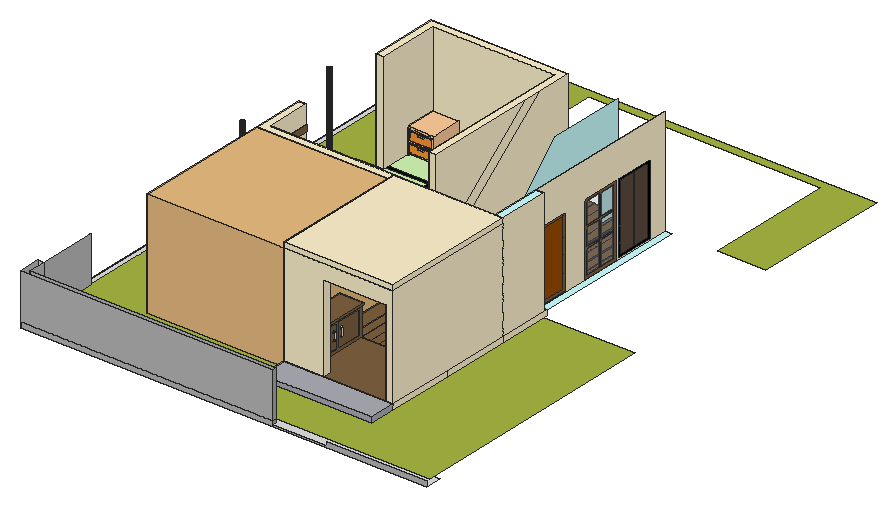
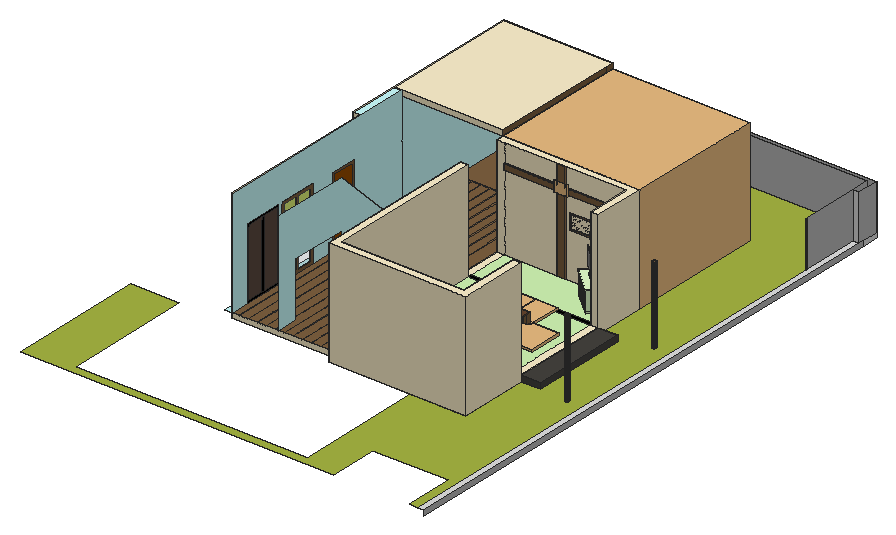
# SketchUp Ruby script. Lengths in inches.
U = 1.inch
M = Sketchup.active_model
def pt(a) = Geom::Point3d.new(a.map { |v| v * U })
def face(e, loops, mat)
  f = e.add_face(loops[0].map { |a| pt(a) })
  loops[1..].each { |l| e.add_face(l.map { |a| pt(a) }).erase! }
  f.material = f.back_material = mat if mat
  f
end
# faces: each face lists its corners as indices into pts; further lists are holes
def faces(e, pts, list, mat = nil) = list.each { |f| face(e, (f[0].is_a?(Array) ? f : [f]).map { |l| l.map { |i| pts[i] } }, mat) }
# xy, xz, yz: faces in a plane at the given z, y or x. An outline is a flat list of corners, or four numbers for a rectangle; further outlines are holes
def ring(l) = l.size == 4 ? [[l[0], l[1]], [l[2], l[1]], [l[2], l[3]], [l[0], l[3]]] : l.each_slice(2).to_a
def flat(e, list, mat, &to3) = list.each { |f| face(e, (f[0].is_a?(Array) ? f : [f]).map { |l| ring(l).map { |u, v| to3.(u, v) } }, mat) }
def xy(e, z, list, mat = nil) = flat(e, list, mat) { |x, y| [x, y, z] }
def xz(e, y, list, mat = nil) = flat(e, list, mat) { |x, z| [x, y, z] }
def yz(e, x, list, mat = nil) = flat(e, list, mat) { |y, z| [x, y, z] }
def lines(e, pts, list) = list.each { |a, b| e.add_line(pt(pts[a]), pt(pts[b])) }
# prism: a flat outline (further loops are holes) pulled along v
def prism(e, loops, v, mat = nil)
  f = face(e, loops, mat); d = Geom::Vector3d.new(v.map { |x| x * U })
  f.pushpull(f.normal.samedirection?(d) ? d.length : -d.length)
end
def box(e, o, s, mat = nil) = prism(e, [[o, [o[0] + s[0], o[1], o[2]], [o[0] + s[0], o[1] + s[1], o[2]], [o[0], o[1] + s[1], o[2]]]], [0, 0, s[2]], mat)
def at(x, y, z, deg = 0) = Geom::Transformation.translation(pt([x, y, z])) * Geom::Transformation.rotation(ORIGIN, Z_AXIS, deg.degrees)
def axes(o, x, y, z) = Geom::Transformation.new([*x, 0, *y, 0, *z, 0, *pt(o).to_a, 1])
def part(name) = M.definitions.add(name)
# library, detail: a bought-in or finely detailed component or shape, given as its bounding box
def library(name, o, s) = part(name).tap { |d| box(d.entities, o, s) }
def detail(e, o, s) = box(e.add_group.entities, o, s)
def put(e, d, t, mat = nil) = e.add_instance(d, t).tap { |i| i.material = mat if mat }
def group(e, t, mat = nil) = e.add_group.tap { |g| g.transformation = t; g.material = mat if mat }.entities
root = M.entities
M.materials.add("A02_Rose_Quartz").color = [255, 153, 153]
M.materials.add("A04_Scarlet_Glow").color = [255, 49, 49]
M.materials.add("Black_Lines_1_1K").color = [210, 247, 181]
M.materials.add("Brick_Stack_Bond_2K2").color = [186, 186, 186]
M.materials.add("C02_Golden_Beige").color = [255, 205, 155]
M.materials.add("C04_Amber_Sunshine").color = [255, 152, 49]
M.materials.add("C07_Caramel_Shine").color = [153, 76, 0]
M.materials.add("D01_Frost_White").color = [255, 242, 206]
M.materials.add("F01_Seafoam_Drift").color = [229, 255, 204]
M.materials.add("Fabric_13_1K").color = [243, 117, 128]
M.materials["Fabric_13_1K"].alpha = 0.97
M.materials.add("Glass_Basic_1").color = [161, 173, 186]
M.materials["Glass_Basic_1"].alpha = 0.25
M.materials.add("Glass_Mirror_01").color = [185, 185, 185]
M.materials["Glass_Mirror_01"].alpha = 0.58
M.materials.add("H01_Misty_Ice1").color = [204, 255, 255]
M.materials.add("M00_Soft_Cloud").color = [255, 255, 255]
M.materials.add("M01_Silver_Fog").color = [224, 224, 224]
M.materials.add("M03_Pewter_Shine").color = [168, 168, 168]
M.materials.add("M04_Stone_Frost").color = [142, 142, 142]
M.materials.add("M07_Charcoal_Gleam").color = [58, 58, 58]
M.materials.add("M09_Shadow_Night").color = [0, 0, 0]
M.materials.add("Marble_20_1K").color = [172, 173, 182]
M.materials.add("Metal_06_1K").color = [238, 236, 231]
M.materials.add("Metal_10_1K").color = [196, 175, 123]
M.materials.add("Plywood_01_1K").color = [125, 96, 64]
M.materials.add("Soil_04_1K").color = [167, 182, 67]
M.materials.add("Wood_Floor_01_1K1").color = [146, 111, 76]
M.materials.add("Wood_Floor_12_1K").color = [92, 75, 65]
M.materials.add("Wood_Planks_01_1K1").color = [69, 67, 63]
M.materials.add("Wood_Veneer_15_1K").color = [103, 69, 45]
c1 = part("Group\#52")
box(c1.entities,[0,0,0],[1.5,12,12.52])
c2 = library("Group\#7",[0,0,0],[162,162,126])
c3 = library("Group\#106",[0,0,0],[9.9375,0.625,10.1875])
c4 = part("Group\#101")
box(c4.entities,[0,0,0],[6,6,17.625],"Plywood_01_1K")
c5 = library("Group\#105",[0,0,-6.9375],[37.03,37.03,8.9375])
c6 = part("Group\#134")
box(c6.entities,[0,0,0],[10.25,2.1875,0.25],"Metal_10_1K")
c7 = library("Group\#86",[-0.0625,-4,0],[20.0625,57.25,28.48])
c8 = part("Group\#46")
detail(c8.entities,[0,0,0],[3.47,3.07,3.07])
c9 = part("Group\#153")
xy(c9.entities,0,[[0,-9.8125,1.5625,-7.9375],[0,-0.1875,1.5625,0],[0,0,1.5625,1.5625]],"Metal_06_1K")
xy(c9.entities,0.29,[[0,-9.8125,1.5625,-8.1875]],"Metal_06_1K")
xy(c9.entities,0.3125,[[0,0,1.5625,1.5625]],"Metal_06_1K")
xy(c9.entities,2.125,[[0,-7.9375,1.5625,-0.1875],[0,-0.1875,1.5625,0]],"Metal_06_1K")
xy(c9.entities,2.375,[[0,-8.1875,1.5625,-7.9375],[0,-7.9375,1.5625,0]],"Metal_06_1K")
xz(c9.entities,-9.8125,[[0,0,1.5625,0.29]],"Metal_06_1K")
xz(c9.entities,-8.1875,[[0,0.29,1.5625,2.375]],"Metal_06_1K")
xz(c9.entities,-7.9375,[[0,0,1.5625,2.125],[0,2.125,1.5625,2.375]],"Metal_06_1K")
xz(c9.entities,-0.1875,[[0,0,1.5625,2.125]],"Metal_06_1K")
xz(c9.entities,0,[[0,0,1.5625,0.3125],[0,0.3125,1.5625,2.125],[0,2.125,1.5625,2.375]],"Metal_06_1K")
xz(c9.entities,1.5625,[[0,0,1.5625,0.3125]],"Metal_06_1K")
yz(c9.entities,0,[[-9.8125,0,-9.8125,0.29,-8.1875,0.29,-8.1875,2.375,-7.9375,2.375,-7.9375,0],[-0.1875,0,0,2.125],[0,0,1.5625,0.3125],[-7.9375,2.125,0,2.375]],"Metal_06_1K")
yz(c9.entities,1.5625,[[-9.8125,0,-7.9375,0,-7.9375,2.375,-8.1875,2.375,-8.1875,0.29,-9.8125,0.29],[-0.1875,0,0,2.125],[0,0,1.5625,0.3125],[-7.9375,2.125,0,2.375]],"Metal_06_1K")
xy(root,6,[[1567.75,129.625,2047.75,149.6875]],"M01_Silver_Fog")
xy(root,12,[[1648.75,215.6875,1801.75,215.6875,1801.75,224.6875,1657.75,224.6875,1657.75,368.6875,1648.75,368.6875],[1801.75,215.6875,1810.75,215.6875,1810.75,580.6875,1876.75,580.6875,1876.75,590.6875,1810.75,590.6875,1810.75,635.6875,1657.75,635.6875,1657.75,626.6875,1801.75,626.6875,1801.75,377.6875,1648.75,377.6875,1648.75,368.6875,1801.75,368.6875],[1657.75,224.6875,1801.75,368.6875],[1810.75,224.6875,1930.75,368.6875],[1648.75,377.6875,1657.75,635.6875],
  [1657.75,377.6875,1801.75,626.6875]],"Brick_Stack_Bond_2K2")
xy(root,12,[[1567.75,129.625,1574.75,149.6875],[1574.75,129.625,1865.79,134.375],[1567.75,149.6875,1574.75,155.6875],[1567.75,155.6875,1567.75,798.625,1574.3125,798.625,1574.3125,224.6875,1574.75,224.6875,1574.75,155.6875]],"M01_Silver_Fog")
xy(root,12,[[1574.75,134.375,2047.75,134.375,2047.75,437.6875,1939.75,437.6875,1939.75,215.6875,1648.75,215.6875,1648.75,635.6875,1712.6875,635.6875,1712.6875,788.6875,1986.9375,788.6875,1986.9375,635.6875,2044.5625,635.6875,2044.5625,798.625,1674.5,798.625,1674.5,740.6875,1584.5,740.6875,1584.5,798.625,1574.3125,798.625,1574.3125,224.6875,1574.75,224.6875]],"Soil_04_1K")
xy(root,18,[[1876.75,440.3125,1882.75,533.5]],"Brick_Stack_Bond_2K2")
xy(root,18,[[1876.75,435.3125,1882.75,440.3125]],"Wood_Floor_12_1K")
xz(root,129.625,[[1567.75,6,2047.75,6,2047.75,12,1929.96,12,1929.96,7.5,1865.79,7.5,1865.79,12,1567.75,12],[1567.75,12,1865.79,66]],"Brick_Stack_Bond_2K2")
xz(root,134.375,[[1574.75,12,1865.79,66]],"Brick_Stack_Bond_2K2")
xz(root,155.6875,[[1567.75,12,1574.75,66]],"M01_Silver_Fog")
xz(root,224.6875,[[1574.3125,12,1574.75,66]],"M01_Silver_Fog")
xz(root,435.3125,[[1876.75,18,1882.75,45.8125]],"Wood_Floor_12_1K")
yz(root,1567.75,[[149.6875,6,798.625,12],[129.625,12,155.6875,66]],"Brick_Stack_Bond_2K2")
yz(root,1567.75,[[129.625,6,149.6875,12]],"M01_Silver_Fog")
yz(root,1574.75,[[134.375,12,155.6875,66],[155.6875,12,224.6875,66]],"Brick_Stack_Bond_2K2")
yz(root,1865.79,[[129.625,7.5,134.375,12],[129.625,12,134.375,66]],"M03_Pewter_Shine")
yz(root,1876.75,[[440.3125,18,440.3125,45.8125,533.5,139,626.6875,139,626.6875,18,602.25,18,602.25,82.875,533.5,82.875,533.5,18]],"H01_Misty_Ice1")
yz(root,1876.75,[[435.3125,18,435.3125,45.77,437.79,43.29,440.3125,45.8125,440.3125,18]],"Wood_Floor_12_1K")
g1 = group(root,at(1590.43,424.46,12))
xy(g1,0,[[2.1875,0,1.62,0.07,1.09,0.29,0.64,0.64,0.29,1.09,0.07,1.62,0,2.1875,0.07,2.75,0.29,3.28,0.64,3.73,1.09,4.08,1.62,4.3,2.1875,4.375,2.75,4.3,3.28,4.08,3.73,3.73,4.08,3.28,4.3,2.75,4.375,2.1875,4.3,1.62,4.08,1.09,3.73,0.64,3.28,0.29,2.75,0.07]],"Metal_06_1K")
xy(g1,91.125,[[2.1875,0,2.75,0.07,3.28,0.29,3.73,0.64,4.08,1.09,4.3,1.62,4.375,2.1875,4.3,2.75,4.08,3.28,3.73,3.73,3.28,4.08,2.75,4.3,2.1875,4.375,1.62,4.3,1.09,4.08,0.64,3.73,0.29,3.28,0.07,2.75,0,2.1875,0.07,1.62,0.29,1.09,0.64,0.64,1.09,0.29,1.62,0.07]],"Plywood_01_1K")
p = [[1.62,0.07,0],[2.1875,0,0],[2.1875,0,91.125],[1.62,0.07,91.125],[2.75,0.07,0],[2.75,0.07,91.125],
  [1.09,0.29,0],[1.09,0.29,91.125],[3.28,0.29,0],[3.28,0.29,91.125],[0.64,0.64,0],[0.64,0.64,91.125],
  [3.73,0.64,0],[3.73,0.64,91.125],[0.29,1.09,0],[0.29,1.09,91.125],[4.08,1.09,0],[4.08,1.09,91.125],
  [0.07,1.62,0],[0.07,1.62,91.125],[4.3,1.62,0],[4.3,1.62,91.125],[0,2.1875,0],[0,2.1875,91.125],
  [4.375,2.1875,0],[4.375,2.1875,91.125],[0.07,2.75,0],[0.07,2.75,91.125],[4.3,2.75,0],[4.3,2.75,91.125],
  [0.29,3.28,0],[0.29,3.28,91.125],[4.08,3.28,0],[4.08,3.28,91.125],[0.64,3.73,0],[0.64,3.73,91.125],
  [3.73,3.73,0],[3.73,3.73,91.125],[1.09,4.08,0],[1.09,4.08,91.125],[3.28,4.08,0],[3.28,4.08,91.125],
  [1.62,4.3,0],[1.62,4.3,91.125],[2.75,4.3,0],[2.75,4.3,91.125],[2.1875,4.375,0],[2.1875,4.375,91.125]]
faces(g1,p,[[0,1,2,3],[1,4,5,2],[6,0,3,7],[4,8,9,5],[10,6,7,11],[8,12,13,9],[14,10,11,15],[12,16,17,13],
  [18,14,15,19],[16,20,21,17],[22,18,19,23],[20,24,25,21],[26,22,23,27],[24,28,29,25],[30,26,27,31],[28,32,33,29],
  [34,30,31,35],[32,36,37,33],[38,34,35,39],[36,40,41,37],[42,38,39,43],[40,44,45,41],[46,42,43,47],[44,46,47,45]],"Plywood_01_1K")
g2 = group(root,at(1590.43,552.78,12),"Plywood_01_1K")
xy(g2,0,[[2.1875,0,1.62,0.07,1.09,0.29,0.64,0.64,0.29,1.09,0.07,1.62,0,2.1875,0.07,2.75,0.29,3.28,0.64,3.73,1.09,4.08,1.62,4.3,2.1875,4.375,2.75,4.3,3.28,4.08,3.73,3.73,4.08,3.28,4.3,2.75,4.375,2.1875,4.3,1.62,4.08,1.09,3.73,0.64,3.28,0.29,2.75,0.07]],"Metal_06_1K")
xy(g2,91.125,[[2.1875,0,2.75,0.07,3.28,0.29,3.73,0.64,4.08,1.09,4.3,1.62,4.375,2.1875,4.3,2.75,4.08,3.28,3.73,3.73,3.28,4.08,2.75,4.3,2.1875,4.375,1.62,4.3,1.09,4.08,0.64,3.73,0.29,3.28,0.07,2.75,0,2.1875,0.07,1.62,0.29,1.09,0.64,0.64,1.09,0.29,1.62,0.07]],"Plywood_01_1K")
p = [[1.62,0.07,0],[2.1875,0,0],[2.1875,0,91.125],[1.62,0.07,91.125],[2.75,0.07,0],[2.75,0.07,91.125],
  [1.09,0.29,0],[1.09,0.29,91.125],[3.28,0.29,0],[3.28,0.29,91.125],[0.64,0.64,0],[0.64,0.64,91.125],
  [3.73,0.64,0],[3.73,0.64,91.125],[0.29,1.09,0],[0.29,1.09,91.125],[4.08,1.09,0],[4.08,1.09,91.125],
  [0.07,1.62,0],[0.07,1.62,91.125],[4.3,1.62,0],[4.3,1.62,91.125],[0,2.1875,0],[0,2.1875,91.125],
  [4.375,2.1875,0],[4.375,2.1875,91.125],[0.07,2.75,0],[0.07,2.75,91.125],[4.3,2.75,0],[4.3,2.75,91.125],
  [0.29,3.28,0],[0.29,3.28,91.125],[4.08,3.28,0],[4.08,3.28,91.125],[0.64,3.73,0],[0.64,3.73,91.125],
  [3.73,3.73,0],[3.73,3.73,91.125],[1.09,4.08,0],[1.09,4.08,91.125],[3.28,4.08,0],[3.28,4.08,91.125],
  [1.62,4.3,0],[1.62,4.3,91.125],[2.75,4.3,0],[2.75,4.3,91.125],[2.1875,4.375,0],[2.1875,4.375,91.125]]
faces(g2,p,[[0,1,2,3],[1,4,5,2],[6,0,3,7],[4,8,9,5],[10,6,7,11],[8,12,13,9],[14,10,11,15],[12,16,17,13],
  [18,14,15,19],[16,20,21,17],[22,18,19,23],[20,24,25,21],[26,22,23,27],[24,28,29,25],[30,26,27,31],[28,32,33,29],
  [34,30,31,35],[32,36,37,33],[38,34,35,39],[36,40,41,37],[42,38,39,43],[40,44,45,41],[46,42,43,47],[44,46,47,45]],"Plywood_01_1K")
g3 = group(root,at(1625.5625,453.84,12))
xy(g3,0,[[0,-14.13,23.1875,99.9]],"Plywood_01_1K")
xy(g3,7,[[0,-14.13,23.1875,99.9]],"Wood_Planks_01_1K1")
xz(g3,-14.13,[[0,0,23.1875,7]],"Wood_Planks_01_1K1")
xz(g3,99.9,[[0,0,23.1875,7]],"Wood_Planks_01_1K1")
yz(g3,0,[[-14.13,0,99.9,7]],"Wood_Planks_01_1K1")
yz(g3,23.1875,[[-14.13,0,99.9,7]],"Plywood_01_1K")
g4 = group(root,at(1660.81,354.75,18.1))
g5 = group(g4,at(0,0,16.54))
box(g5,[0,0,0],[65.15,12,1.64],"Wood_Floor_12_1K")
g6 = group(g4,at(0,0,18.18),"Wood_Floor_12_1K")
box(g6,[0,0,0],[1.5,12,14.9])
g7 = group(g4,at(0,0,33.08))
box(g7,[0,0,0],[65.15,12,1.64],"Wood_Floor_12_1K")
put(g4,c1,axes([63.65,0,18.18],[1,0,0],[0,1,0],[0,0,1.19]),"Wood_Floor_12_1K")
put(g4,c1,axes([0,0,1.64],[1,0,0],[0,1,0],[0,0,1.19]),"Wood_Floor_12_1K")
g8 = group(g4,at(0,13.5,0))
box(g8,[0,-1.5,0],[65.15,1.5,34.72],"Wood_Floor_12_1K")
g9 = group(g4,at(0,0,0))
box(g9,[0,0,0],[65.15,12,1.64],"Wood_Floor_12_1K")
put(g4,c1,axes([63.65,0,1.64],[1,0,0],[0,1,0],[0,0,1.19]),"Wood_Floor_12_1K")
g10 = group(root,at(1667.95,239.89,18),"Brick_Stack_Bond_2K2")
xy(g10,0,[[[0,0,108.22,93.41],[8,6.84,100.22,86.57]]],"Fabric_13_1K")
xy(g10,1,[[[8,6.84,100.22,86.57],[11.88,10.15,96.34,83.26]],[[18.66,15.95,89.56,77.46],[21.31,18.21,86.91,75.2]]],"A04_Scarlet_Glow")
xy(g10,1,[[[0,0,108.22,93.41],[8,6.84,100.22,86.57]],[[11.88,10.15,96.34,83.26],[18.66,15.95,89.56,77.46]],[21.31,18.21,86.91,75.2]],"C02_Golden_Beige")
xz(g10,0,[[0,0,108.22,1]],"Fabric_13_1K")
xz(g10,6.84,[[8,0,100.22,1]],"Fabric_13_1K")
xz(g10,86.57,[[8,0,100.22,1]],"Fabric_13_1K")
xz(g10,93.41,[[0,0,108.22,1]],"Fabric_13_1K")
yz(g10,0,[[0,0,93.41,1]],"Fabric_13_1K")
yz(g10,8,[[6.84,0,86.57,1]],"Fabric_13_1K")
yz(g10,100.22,[[6.84,0,86.57,1]],"Fabric_13_1K")
yz(g10,108.22,[[0,0,93.41,1]],"Fabric_13_1K")
put(root,c2,at(1648.75,215.6875,12),"D01_Frost_White")
g11 = group(root,at(1657.75,368.6875,18.1),"Brick_Stack_Bond_2K2")
xy(g11,0,[[0,-0.4375,144,0]],"Wood_Floor_01_1K1")
xy(g11,5.17,[[0,-0.4375,144,0]],"Wood_Floor_01_1K1")
xz(g11,-0.4375,[[0,0,144,5.17]],"Plywood_01_1K")
xz(g11,0,[[0,0,144,5.17]],"Wood_Floor_01_1K1")
yz(g11,0,[[-0.4375,0,0,5.17]],"Wood_Floor_01_1K1")
yz(g11,144,[[-0.4375,0,0,5.17]],"Wood_Floor_01_1K1")
g12 = group(root,at(1657.75,377.6875,12),"D01_Frost_White")
xy(g12,0,[[-9,0,153,258]],"D01_Frost_White")
xy(g12,7,[[144,9,153,62.625],[-9,62.02,0,176.05]],"D01_Frost_White")
xy(g12,126,[[-9,0,153,0,153,9,0,9,0,62.02,-9,62.02],[144,62.625,153,62.625,153,194.7,153.375,194.7,153.375,213.98,153,213.98,153,258,-9,258,-9,176.05,0,176.05,0,249,144,249]],"D01_Frost_White")
xz(g12,0,[[-9,0,144,126],[144,0,153,126]],"D01_Frost_White")
xz(g12,9,[[0,7,144,126],[144,7,153,126]],"D01_Frost_White")
xz(g12,62.02,[[-9,7,0,126]],"D01_Frost_White")
xz(g12,62.625,[[144,7,153,126]],"D01_Frost_White")
xz(g12,176.05,[[-9,7,0,126]],"D01_Frost_White")
xz(g12,249,[[0,7,144,126]],"D01_Frost_White")
xz(g12,258,[[-9,0,153,126]],"D01_Frost_White")
yz(g12,-9,[[0,0,0,126,62.02,126,62.02,7,176.05,7,176.05,126,258,126,258,0]],"D01_Frost_White")
yz(g12,0,[[9,7,62.02,126],[176.05,7,249,126]],"D01_Frost_White")
yz(g12,144,[[62.625,7,249,126]],"D01_Frost_White")
yz(g12,153,[[0,0,258,0,258,126,213.98,126,63.04,6,62.625,21,62.625,7,9,7,9,126,0,126],[62.625,21,194.7,126,62.625,126]],"D01_Frost_White")
yz(g12,153.375,[[63.04,6,213.98,126,194.7,126,62.625,21]],"D01_Frost_White")
p = [[153,62.625,21],[153,63.04,6],[153.375,63.04,6],[153.375,62.625,21],[153,213.98,126],[153.375,213.98,126],
  [153,194.7,126],[153.375,194.7,126]]
faces(g12,p,[[0,1,2,3],[1,4,5,2],[6,0,3,7]],"D01_Frost_White")
g13 = group(g12,at(0,9,7),"Wood_Floor_01_1K1")
xy(g13,0,[[71.8125,0,81.0625,1.1]])
xy(g13,90.4375,[[0,0,0,53.02,1.02,53.02,1.02,1.1,71.8125,1.1,71.8125,0],[81.0625,0,144,1.1]])
xy(g13,97.0625,[[81.0625,0,144,1.1]])
xy(g13,97.1875,[[0,0,71.8125,0,71.8125,1.1,1.02,1.1,1.02,53.02,0,53.02]])
xy(g13,119,[[71.8125,0,81.0625,1.1]])
xz(g13,0,[[71.8125,0,81.0625,0,81.0625,90.4375,144,90.4375,144,97.0625,81.0625,97.0625,81.0625,119,71.8125,119,71.8125,97.1875,0,97.1875,0,90.4375,71.8125,90.4375]])
xz(g13,1.1,[[71.8125,0,71.8125,90.4375,1.02,90.4375,1.02,97.1875,71.8125,97.1875,71.8125,119,81.0625,119,81.0625,97.0625,144,97.0625,144,90.4375,81.0625,90.4375,81.0625,0]],"Plywood_01_1K")
xz(g13,53.02,[[0,90.4375,1.02,97.1875]],"Plywood_01_1K")
yz(g13,0,[[0,90.4375,53.02,97.1875]])
yz(g13,1.02,[[1.1,90.4375,53.02,97.1875]],"Plywood_01_1K")
yz(g13,71.8125,[[0,0,1.1,90.4375],[0,97.1875,1.1,119]])
yz(g13,81.0625,[[0,0,1.1,90.4375],[0,97.0625,1.1,119]])
yz(g13,144,[[0,90.4375,1.1,97.0625]])
put(g12,c3,axes([68.41,10.1,95.33],[1.6244,0,0],[0,1,0],[0,0,1.27401]))
g14 = group(g12,at(66.47,9,60.6875))
xy(g14,0,[[-25.9375,0,0,0.79]],"Plywood_01_1K")
xy(g14,1.27,[[-24.67,0,-1.27,0.79]],"Plywood_01_1K")
xy(g14,17.29,[[-24.67,0,-1.27,0.79]],"Plywood_01_1K")
xy(g14,18.5625,[[-25.9375,0,0,0.79]],"Plywood_01_1K")
xz(g14,0,[[[-25.9375,0,0,18.5625],[-24.67,1.27,-1.27,17.29]],[-24.67,1.27,-1.27,17.29]],"Plywood_01_1K")
xz(g14,0.79,[[[-25.9375,0,0,18.5625],[-24.67,1.27,-1.27,17.29]]],"Plywood_01_1K")
yz(g14,-25.9375,[[0,0,0.79,18.5625]],"Plywood_01_1K")
yz(g14,-24.67,[[0,1.27,0.79,17.29]],"Plywood_01_1K")
yz(g14,-1.27,[[0,1.27,0.79,17.29]],"Plywood_01_1K")
yz(g14,0,[[0,0,0.79,18.5625]],"Plywood_01_1K")
g15 = group(g12,at(0,9,7))
g16 = group(g15,at(0,0,0))
g17 = group(g16,at(0.98,2.41,0))
xy(g17,0,[[28.45,-1.77,0,23.17,15.04,37.4,42.39,13.41]])
xy(g17,2.06,[[28.45,-1.77,0,23.17,15.04,37.4,42.39,13.41]])
xy(g17,4.35,[[40.72,14.87,28.72,25.4,28.83,25.52,40.83,14.99]],"M00_Soft_Cloud")
xy(g17,4.35,[[28.72,25.4,16.71,35.93,16.82,36.05,28.83,25.52]],"M07_Charcoal_Gleam")
xy(g17,4.76,[[40.43,15.13,40.54,15.25,28.92,25.4375,28.8125,25.32],[28.58,25.52,28.69,25.64,17.12,35.79,17.01,35.67]],"M07_Charcoal_Gleam")
xy(g17,22.77,[[40.43,15.13,28.8125,25.32,28.92,25.4375,40.54,15.25],[28.58,25.52,17.01,35.67,17.12,35.79,28.69,25.64]],"M07_Charcoal_Gleam")
xy(g17,23.18,[[40.72,14.87,40.83,14.99,28.83,25.52,28.72,25.4],[28.72,25.4,28.83,25.52,16.82,36.05,16.71,35.93]],"M07_Charcoal_Gleam")
xy(g17,25.48,[[28.45,-1.77,0,23.17,15.04,37.4,15.61,36.9,42.39,13.41]])
xy(g17,25.48,[[29.17,-2.41,28.45,-1.77,42.39,13.41,15.61,36.9,16.37,37.73,43.88,13.6],[0,23.17,-0.98,24.17,14.02,38.36,13.99,38.32,15.04,37.4],[15.61,36.9,15.04,37.4,14.06,38.39,14.02,38.36,14.75,39.15,16.37,37.73],[15.04,37.4,13.99,38.32,14.02,38.36,14.06,38.39]],"F01_Seafoam_Drift")
xy(g17,26.53,[[29.17,-2.41,43.88,13.6,14.75,39.15,14.02,38.36,-0.98,24.17,0,23.17]],"F01_Seafoam_Drift")
p = [[0,23.17,0],[28.45,-1.77,0],[28.45,-1.77,2.06],[0,23.17,2.06],[42.39,13.41,0],[42.39,13.41,2.06],
  [15.04,37.4,0],[15.04,37.4,2.06],[28.45,-1.77,25.48],[0,23.17,25.48],[42.39,13.41,25.48],[15.04,37.4,25.48],
  [15.61,36.9,25.48],[28.72,25.4,4.35],[40.72,14.87,4.35],[40.72,14.87,23.18],[28.72,25.4,23.18],[16.71,35.93,23.18],
  [16.71,35.93,4.35],[40.83,14.99,4.35],[40.83,14.99,23.18],[28.83,25.52,4.35],[16.82,36.05,4.35],[16.82,36.05,23.18],
  [28.83,25.52,23.18],[28.92,25.4375,4.76],[40.54,15.25,4.76],[40.54,15.25,22.77],[28.92,25.4375,22.77],[28.69,25.64,22.77],
  [17.12,35.79,22.77],[17.12,35.79,4.76],[28.69,25.64,4.76],[40.43,15.13,4.76],[28.8125,25.32,4.76],[28.8125,25.32,22.77],
  [40.43,15.13,22.77],[17.01,35.67,22.77],[28.58,25.52,22.77],[28.58,25.52,4.76],[17.01,35.67,4.76],[29.17,-2.41,25.48],
  [29.17,-2.41,26.53],[0,23.17,26.53],[43.88,13.6,25.48],[43.88,13.6,26.53],[16.37,37.73,25.48],[14.75,39.15,25.48],
  [14.75,39.15,26.53],[-0.98,24.17,26.53],[-0.98,24.17,25.48],[14.02,38.36,25.48],[14.02,38.36,26.53],[14.06,38.39,26.53],
  [14.06,38.39,25.48],[13.99,38.32,25.48],[13.99,38.32,26.53]]
faces(g17,p,[[0,1,2,3],[3,2,8,9],[9,8,41,42,43],[9,43,49,50]])
faces(g17,p,[[1,4,5,2],[4,6,7,5],[6,0,3,7],[8,2,5,10],[[5,7,11,12,10],[13,14,15,16,17,18]],[7,3,9,11],[41,44,45,42],[44,46,47,48,45],
  [51,50,49,52,53,54],[55,56,52,48,47,51]],"F01_Seafoam_Drift")
faces(g17,p,[[15,14,19,20],[[19,21,22,23,24,20],[25,26,27,28],[29,30,31,32]],[18,17,23,22],[33,36,27,26],[35,34,25,28],[39,38,29,32],[37,40,31,30]],"M07_Charcoal_Gleam")
faces(g17,p,[[33,34,35,36],[37,38,39,40]],"M00_Soft_Cloud")
g18 = group(g16,at(17.61,25.76,26.53),"M09_Shadow_Night")
xy(g18,0,[[12.06,-10.58,0,0,1.38,1.5,13.4375,-9.07]])
xy(g18,0.95,[[12.06,-10.58,13.4375,-9.07,1.38,1.5,0,0]])
p = [[0,0,0],[12.06,-10.58,0],[12.06,-10.58,0.95],[0,0,0.95],[13.4375,-9.07,0],[13.4375,-9.07,0.95],
  [1.38,1.5,0],[1.38,1.5,0.95],[1.57,1.34,0.69],[1.57,1.34,0.25],[13.25,-8.91,0.25],[13.25,-8.91,0.69]]
faces(g18,p,[[0,1,2,3],[1,4,5,2],[[4,6,7,5],[8,9,10,11]],[6,0,3,7]])
faces(g18,p,[[9,8,11,10]],"M04_Stone_Frost")
g19 = group(g18,at(3.51,-2.17,0.95))
prism(g19,[[[0.45,0.49,0],[6.08,-4.44,0],[5.63,-4.9375,0],[0,0,0]]],[0,0,3.56])
g20 = group(g18,at(3.51,-2.17,4.51))
xy(g20,0,[[16.88,-14.8,-10.36,9.08,-9.91,9.58,17.33,-14.3125]])
xy(g20,20.36,[[16.88,-14.8,17.33,-14.3125,-9.91,9.58,-10.36,9.08]])
p = [[-10.36,9.08,0],[16.88,-14.8,0],[16.88,-14.8,20.36],[-10.36,9.08,20.36],[17.33,-14.3125,0],[17.33,-14.3125,20.36],
  [-9.91,9.58,0],[-9.91,9.58,20.36],[-9.23,8.98,19.29],[-9.23,8.98,0.67],[16.34,-13.44,0.67],[16.34,-13.44,19.29]]
faces(g20,p,[[0,1,2,3],[1,4,5,2],[[6,7,5,4],[8,9,10,11]],[6,0,3,7]])
faces(g20,p,[[8,11,10,9]],"Glass_Mirror_01")
g21 = group(g15,at(31.11,26.25,14.27))
prism(g21,[[[0.37,0,0],[0,0.33,0],[0.08,0.43,0],[0.46,0.09,0]]],[0,0,3.8125],"Metal_06_1K")
g22 = group(g15,at(28.24,28.77,14.1875))
prism(g22,[[[0.37,0,0],[0,0.33,0],[0.08,0.43,0],[0.46,0.09,0]]],[0,0,3.8125],"Metal_06_1K")
g23 = group(g12,at(0,9,7))
xy(g23,0,[[0,0,144,49.09],[0,53.34,48.81,171.05],[53.6,53.34,107.2,171.05],[111.37,53.34,144,171.05],[0,174.98,72,240],
  [76.1,174.98,144,240]],"Black_Lines_1_1K")
xy(g23,0,[[[0,49.09,144,49.09,144,53.34,111.37,53.34,111.37,171.05,144,171.05,144,174.98,76.1,174.98,76.1,240,72,240,72,174.98,0,174.98,0,171.05,48.81,171.05,48.81,53.34,0,53.34],[53.6,53.34,107.2,171.05]]],"M09_Shadow_Night")
g24 = group(g23,at(44.43,87.51,0))
put(g24,c4,axes([0,0,0],[0.77733,0,0],[0,0.72,0],[0,0,0.66]))
put(g24,c4,axes([58.11,0,0],[0.77733,0,0],[0,0.72,0],[0,0,0.66]))
put(g24,c4,axes([58.11,32.89,0],[0.77733,0,0],[0,0.72,0],[0,0,0.66]))
put(g24,c4,axes([0,32.89,0],[0.77733,0,0],[0,0.72,0],[0,0,0.66]))
g25 = group(g24,at(0,0,11.63))
box(g25,[0,0,0],[62.77,37.21,1.32],"Wood_Veneer_15_1K")
put(g23,c5,axes([69.26,118.59,0],[1.1235,0,0],[0,1.09356,0],[0,0,1]))
put(g23,c5,axes([43.26,118.59,0],[1.1235,0,0],[0,1.09356,0],[0,0,1]))
put(g23,c5,axes([97.21,84.52,0],[1.1235,0,0],[0,1.09356,0],[0,0,1]))
put(g23,c5,axes([10.22,86.27,0],[1.1235,0,0],[0,1.09356,0],[0,0,1]))
put(g23,c5,axes([41.43,49.48,0],[1.1235,0,0],[0,1.09356,0],[0,0,1]))
put(g23,c5,axes([67.43,49.48,0],[1.1235,0,0],[0,1.09356,0],[0,0,1]))
g26 = group(g12,at(0,211.6875,7))
xy(g26,0,[[0,0,0,37.3125,30.64,37.3125,30.64,31.32,20.31,31.32,20.31,4.64,2.45,4.64,2.45,0],[28.21,0,30.64,4.64]])
xy(g26,1.36,[[20.31,4.64,30.64,31.32]],"C02_Golden_Beige")
xy(g26,1.4,[[2.45,0,28.21,4.64]],"C02_Golden_Beige")
xy(g26,30.01,[[0,0,30.64,37.3125]],"C02_Golden_Beige")
xz(g26,0,[[[0,0,2.45,0,2.45,1.4,28.21,1.4,28.21,0,30.64,0,30.64,30.01,0,30.01],[1.93,15.4,28.71,27.92],[1.93,2.09,28.71,14.57]]],"C02_Golden_Beige")
xz(g26,0,[[2.17,2.35,28.47,11.95],[2.17,12.1,28.47,14.31],[2.17,15.66,28.47,25.33],[2.17,25.45,28.47,27.66]],"C04_Amber_Sunshine")
xz(g26,0,[[[1.93,2.09,28.71,14.57],[2.17,2.35,28.47,14.31]],[2.17,11.95,28.47,12.1],[1.93,15.4,28.71,15.4,28.71,27.92,1.93,27.92,1.93,25.45,2.17,25.45,2.17,27.66,28.47,27.66,28.47,15.66,2.17,15.66,2.17,25.33,1.93,25.33],[1.93,25.33,2.17,25.45],[2.17,25.33,28.47,25.45]],"M09_Shadow_Night")
xz(g26,4.64,[[2.45,0,20.31,0,20.31,1.36,28.21,1.36,28.21,1.4,2.45,1.4],[20.31,0,28.21,1.36],[28.21,0,30.64,1.36]],"C02_Golden_Beige")
xz(g26,31.32,[[20.31,0,30.64,1.36]],"C02_Golden_Beige")
xz(g26,37.3125,[[0,0,30.64,30.01]])
yz(g26,0,[[0,0,37.3125,30.01]])
yz(g26,2.45,[[0,0,4.64,1.4]],"C02_Golden_Beige")
yz(g26,20.31,[[4.64,0,31.32,1.36]],"C02_Golden_Beige")
yz(g26,28.21,[[0,0,4.64,1.4]],"C02_Golden_Beige")
yz(g26,30.64,[[0,0,4.64,0,4.64,1.36,31.32,1.36,31.32,0,37.3125,0,37.3125,30.01,0,30.01]],"C02_Golden_Beige")
put(g26,c6,axes([12.05,0,9.57],[0.646,0,0],[0,0,0.7],[0,-1,0]))
put(g26,c6,axes([12.05,0,23.4],[0.646,0,0],[0,0,0.7],[0,-1,0]))
put(root,c7,at(1781.65,228.18,18.1),"A02_Rose_Quartz")
g27 = group(root,at(1801.75,224.6875,18.1),"Brick_Stack_Bond_2K2")
box(g27,[-0.1,0,0],[0.1,98.5625,5.17],"Plywood_01_1K")
xy(g27,0,[[-0.1,134.5625,0,143.5625]],"Wood_Floor_01_1K1")
xy(g27,5.17,[[-0.1,134.5625,0,143.5625]],"Wood_Floor_01_1K1")
xz(g27,134.5625,[[-0.1,0,0,5.17]],"Wood_Floor_01_1K1")
xz(g27,143.5625,[[-0.1,0,0,5.17]],"Wood_Floor_01_1K1")
yz(g27,-0.1,[[134.5625,0,143.5625,5.17]],"Plywood_01_1K")
yz(g27,0,[[134.5625,0,143.5625,5.17]],"Wood_Floor_01_1K1")
p = [[0,98.5625,-0.1],[0,98.5625,0],[0,134.5625,0],[0,134.5625,-0.1]]
lines(g27,p,[[0,1],[2,3]])
g28 = group(root,at(1808.06,323.25,18.1))
xy(g28,0,[[2.59,-0.01,-6,0.02,-5.9,36.02,2.69,35.99]],"Wood_Floor_01_1K1")
xy(g28,3,[[0.01,3,0.09,33,-5.91,33.02,-5.99,3.02]],"Plywood_01_1K")
xy(g28,3,[[2.6,2.99,2.68,32.99,0.09,33,0.01,3]],"Wood_Floor_12_1K")
xy(g28,80.9,[[0.01,3,-5.99,3.02,-5.91,33.02,0.09,33]],"Plywood_01_1K")
xy(g28,80.9,[[2.6,2.99,0.01,3,0.09,33,2.68,32.99]],"Wood_Floor_12_1K")
xy(g28,83.9,[[2.59,-0.01,2.69,35.99,-5.9,36.02,-6,0.02]],"Wood_Floor_01_1K1")
p = [[-6,0.02,0],[-6,0.02,83.9],[-5.9,36.02,83.9],[-5.9,36.02,0],[-5.99,3.02,80.9],[-5.99,3.02,3],
  [-5.91,33.02,3],[-5.91,33.02,80.9],[2.59,-0.01,0],[2.59,-0.01,83.9],[2.69,35.99,0],[2.69,35.99,83.9],
  [2.6,2.99,3],[2.6,2.99,80.9],[2.68,32.99,80.9],[2.68,32.99,3],[0.01,3,80.9],[0.01,3,3],
  [0.09,33,3],[0.09,33,80.9]]
faces(g28,p,[[[0,1,2,3],[4,5,6,7]],[0,8,9,1],[2,11,10,3]],"Wood_Floor_01_1K1")
faces(g28,p,[[[9,8,10,11],[12,13,14,15]],[17,16,13,12],[19,18,15,14]],"Wood_Floor_12_1K")
faces(g28,p,[[16,17,5,4],[5,4,7,6],[16,17,18,19],[18,19,7,6]],"Plywood_01_1K")
put(g28,c8,axes([-6.41,27.73,42.96],[0.14,0,0],[0,1,0],[0,0,1]),"Metal_06_1K")
put(g28,c8,axes([0.07,26.88,45.87],[0.14,0,0],[0,1,0],[0,0,1]),"Metal_06_1K")
g29 = group(root,at(1810.75,295.6875,18),"Plywood_01_1K")
box(g29,[0,0,0],[0.3125,27.5625,6.51])
box(g29,[0,63.5625,0],[0.3125,18.4375,6.51])
g30 = group(root,at(1810.75,224.6875,18))
xy(g30,0,[[0,0,27.1,71],[27.1,0,27.54,71]],"Plywood_01_1K")
xy(g30,3,[[27.1,3,27.54,34.5],[27.1,36.5,27.54,68]],"Plywood_01_1K")
xy(g30,31,[[27.1,3,27.54,34.5],[27.1,36.5,27.54,68]],"Plywood_01_1K")
xy(g30,34,[[0,0,27.1,71],[27.1,0,27.54,71],[27.54,0,29.04,71],[0,71,29.04,72.9375]],"Plywood_01_1K")
xy(g30,36,[[0,0,29.04,72.9375]],"Plywood_01_1K")
xz(g30,0,[[0,0,27.1,34],[27.1,0,27.54,34],[0,34,29.04,36]],"Plywood_01_1K")
xz(g30,3,[[27.1,3,27.54,31]],"Plywood_01_1K")
xz(g30,34.5,[[27.1,3,27.54,31]],"Plywood_01_1K")
xz(g30,36.5,[[27.1,3,27.54,31]],"Plywood_01_1K")
xz(g30,68,[[27.1,3,27.54,31]],"Plywood_01_1K")
xz(g30,71,[[0,0,27.1,34],[27.1,0,27.54,34]],"Plywood_01_1K")
xz(g30,72.9375,[[0,34,29.04,36]],"Plywood_01_1K")
yz(g30,0,[[0,0,71,34],[0,34,72.9375,36]],"Plywood_01_1K")
yz(g30,27.1,[[[0,0,71,34],[36.5,3,68,31],[3,3,34.5,31]],[3,3,34.5,31],[36.5,3,68,31]],"Plywood_01_1K")
yz(g30,27.54,[[[0,0,71,34],[36.5,3,68,31],[3,3,34.5,31]]],"Plywood_01_1K")
yz(g30,29.04,[[0,34,72.9375,36]],"Plywood_01_1K")
put(g30,c9,axes([27.1,28.79,23.25],[0,1,0],[0,0,1],[1,0,0]))
put(g30,c9,axes([27.1,39.92,23.25],[0,1,0],[0,0,1],[1,0,0]))
g31 = group(root,at(1810.75,183.5,12),"Marble_20_1K")
box(g31,[0,0,0],[129,32.1875,6])
g32 = group(root,at(1819.75,215.6875,12))
xy(g32,0,[[0,0,120,80],[-9,162,-9,411,111.9375,411,111.9375,226.5,120,226.5,120,162]],"D01_Frost_White")
xy(g32,0,[[-9,0,0,80],[-9,80,0,162]],"Plywood_01_1K")
xy(g32,6,[[111.9375,222,120,226.5]],"D01_Frost_White")
xy(g32,6,[[111,231.25,111.9375,264.625],[111,293,111.9375,338.59],[111,342.5,111.9375,390.6875]],"H01_Misty_Ice1")
xy(g32,6,[[-9,0,7.56,9],[37.5,0,37.5,9,-9,9,-9,80,111,80,111,0],[7.56,0,8.5,9],[8.5,0,18.1,9],[18.1,0,19.07,9],
  [19.07,0,28.65,9],[28.65,0,29.64,9],[29.64,0,37.5,9],[111,0,120,80],[-9,80,7.56,411],
  [7.56,80,8.5,162],[8.5,80,18.1,411],[18.1,80,19.07,162],[19.07,80,28.65,411],[28.65,80,29.64,162],
  [29.64,80,39.19,411],[39.19,80,40.21,162],[40.21,80,49.73,411],[49.73,80,50.78,162],[50.78,80,60.28,411],
  [60.28,80,61.34,162],[61.34,80,70.82,411],[70.82,80,71.91,162],[71.91,80,81.36,411],[81.36,80,82.48,162],
  [82.48,80,91.91,411],[91.91,80,93.05,162],[93.05,80,102.45,411],[102.45,80,103.62,162],[103.62,80,111,411],
  [111,80,120,162]],"Plywood_01_1K")
xy(g32,6,[[7.56,162,8.5,411],[18.1,162,19.07,411],[28.65,162,29.64,411],[39.19,162,40.21,411],[49.73,162,50.78,411],
  [60.28,162,61.34,411],[70.82,162,71.91,411],[81.36,162,82.48,411],[91.91,162,93.05,411],[102.45,162,103.62,411]],"Wood_Planks_01_1K1")
xy(g32,90,[[111,231.25,111.9375,264.625]],"H01_Misty_Ice1")
xy(g32,91,[[111,293,111.9375,338.59],[111,342.5,111.9375,390.6875]],"H01_Misty_Ice1")
xy(g32,108,[[37.5,0,111,9]],"D01_Frost_White")
xy(g32,126,[[-9,0,-9,9,111,9,111,162,120,162,120,0],[-9,9,111,162]],"Plywood_01_1K")
xy(g32,132,[[-9,0,120,162]],"D01_Frost_White")
xy(g32,132,[[111,162,111,411,111.9375,411,111.9375,222,120,222,120,162]],"H01_Misty_Ice1")
xz(g32,0,[[-9,0,120,6],[-9,6,37.5,6,37.5,108,111,108,111,6,120,6,120,126,-9,126],[-9,126,120,132]],"D01_Frost_White")
xz(g32,9,[[-9,6,-9,126,111,126,111,108,37.5,108,37.5,6]],"H01_Misty_Ice1")
xz(g32,80,[[-9,0,120,6]],"D01_Frost_White")
xz(g32,162,[[111,6,120,126]])
xz(g32,162,[[-9,126,111,132]],"D01_Frost_White")
xz(g32,162,[[111,126,120,132]],"H01_Misty_Ice1")
xz(g32,222,[[111.9375,6,120,132]],"D01_Frost_White")
xz(g32,226.5,[[111.9375,0,120,6]],"D01_Frost_White")
xz(g32,231.25,[[111,6,111.9375,90]],"H01_Misty_Ice1")
xz(g32,264.625,[[111,6,111.9375,90]],"H01_Misty_Ice1")
xz(g32,293,[[111,6,111.9375,91]],"H01_Misty_Ice1")
xz(g32,338.59,[[111,6,111.9375,91]],"H01_Misty_Ice1")
xz(g32,342.5,[[111,6,111.9375,91]],"H01_Misty_Ice1")
xz(g32,390.6875,[[111,6,111.9375,91]],"H01_Misty_Ice1")
xz(g32,411,[[-9,0,-9,6,111,6,111,132,111.9375,132,111.9375,0]],"D01_Frost_White")
yz(g32,-9,[[0,6,9,126]],"D01_Frost_White")
yz(g32,-9,[[0,0,80,6],[80,0,411,6],[0,126,9,132],[9,126,162,132]],"Plywood_01_1K")
yz(g32,37.5,[[0,6,9,108]],"D01_Frost_White")
yz(g32,111,[[0,6,9,108]],"D01_Frost_White")
yz(g32,111,[[9,6,162,126],[162,6,231.25,6,231.25,90,264.625,90,264.625,6,293,6,293,91,338.59,91,338.59,6,342.5,6,342.5,91,390.6875,91,390.6875,6,411,6,411,132,162,132]],"H01_Misty_Ice1")
yz(g32,111.9375,[[[226.5,0,411,0,411,132,222,132,222,6,226.5,6],[342.5,6,390.6875,91],[293,6,338.59,91],[231.25,6,264.625,90]]],"D01_Frost_White")
yz(g32,120,[[0,0,80,6],[80,0,162,6],[162,0,226.5,6],[0,6,162,126],[162,6,222,132],
  [0,126,162,132]],"D01_Frost_White")
g33 = group(g32,at(111,162,6))
xy(g33,0,[[0,0,9,249]],"H01_Misty_Ice1")
g34 = group(g32,at(111,231.25,6))
xy(g34,0,[[0,0,0.25,33.375]],"Plywood_01_1K")
xy(g34,3,[[0,3,0.25,30.375]],"Plywood_01_1K")
xy(g34,81,[[0,3,0.25,30.375]],"Plywood_01_1K")
xy(g34,84,[[0,0,0.25,33.375]],"Plywood_01_1K")
xz(g34,0,[[0,0,0.25,84]],"Plywood_01_1K")
xz(g34,3,[[0,3,0.25,81]],"Plywood_01_1K")
xz(g34,30.375,[[0,3,0.25,81]],"Plywood_01_1K")
xz(g34,33.375,[[0,0,0.25,84]],"Plywood_01_1K")
yz(g34,0,[[3,3,30.375,81]],"C07_Caramel_Shine")
yz(g34,0,[[[0,0,33.375,84],[3,3,30.375,81]]],"Plywood_01_1K")
yz(g34,0.25,[[3,3,30.375,81]],"C07_Caramel_Shine")
yz(g34,0.25,[[[0,0,33.375,84],[3,3,30.375,81]]],"Plywood_01_1K")
g35 = group(g32,at(111.9375,293.15,5.92))
xy(g35,0,[[-1.1875,0,0,45.59]],"Plywood_01_1K")
xy(g35,3,[[-1.1875,3,0,21.79],[-1.1875,21.79,0,23.79],[-1.1875,23.79,0,42.59]],"Plywood_01_1K")
xy(g35,31.55,[[-1.1875,3,0,21.79],[-1.1875,23.79,0,42.59]],"Plywood_01_1K")
xy(g35,33.05,[[-1.1875,3,0,21.79],[-1.1875,23.79,0,42.59]],"Plywood_01_1K")
xy(g35,54.24,[[-1.1875,3,0,21.79],[-1.1875,23.79,0,42.59]],"Plywood_01_1K")
xy(g35,55.74,[[-1.1875,3,0,21.79],[-1.1875,23.79,0,42.59]],"Plywood_01_1K")
xy(g35,82,[[-1.1875,3,0,21.79],[-1.1875,21.79,0,23.79],[-1.1875,23.79,0,42.59]],"Plywood_01_1K")
xy(g35,85,[[-1.1875,0,0,45.59]],"Plywood_01_1K")
xz(g35,0,[[-1.1875,0,0,85]],"Plywood_01_1K")
xz(g35,3,[[-1.1875,3,0,31.55],[-1.1875,33.05,0,54.24],[-1.1875,55.74,0,82]],"Plywood_01_1K")
xz(g35,21.79,[[-1.1875,3,0,31.55],[-1.1875,33.05,0,54.24],[-1.1875,55.74,0,82]],"Plywood_01_1K")
xz(g35,23.79,[[-1.1875,3,0,31.55],[-1.1875,33.05,0,54.24],[-1.1875,55.74,0,82]],"Plywood_01_1K")
xz(g35,42.59,[[-1.1875,3,0,31.55],[-1.1875,33.05,0,54.24],[-1.1875,55.74,0,82]],"Plywood_01_1K")
xz(g35,45.59,[[-1.1875,0,0,85]],"Plywood_01_1K")
yz(g35,-1.1875,[[[0,0,45.59,85],[3,3,42.59,3,42.59,31.55,23.79,31.55,23.79,3,21.79,3,21.79,31.55,3,31.55],[3,55.74,21.79,55.74,21.79,82,23.79,82,23.79,55.74,42.59,55.74,42.59,82,3,82],[3,33.05,21.79,54.24],[23.79,33.05,42.59,54.24]]],"Plywood_01_1K")
yz(g35,0,[[3,3,21.79,31.55],[23.79,3,42.59,31.55],[3,33.05,21.79,54.24],[23.79,33.05,42.59,54.24],[3,55.74,21.79,82],
  [23.79,55.74,42.59,82]],"Glass_Basic_1")
yz(g35,0,[[[0,0,45.59,85],[3,3,3,31.55,21.79,31.55,21.79,3,23.79,3,23.79,31.55,42.59,31.55,42.59,3],[3,55.74,3,82,42.59,82,42.59,55.74,23.79,55.74,23.79,82,21.79,82,21.79,55.74],[3,33.05,21.79,54.24],[23.79,33.05,42.59,54.24]]],"Plywood_01_1K")
g36 = group(g32,at(111,342.5,6))
yz(g36,0,[[[0,0,48.1875,85],[3,3,45.1875,82]],[23.09,3,25.09,82]],"M09_Shadow_Night")
yz(g36,0,[[3,3,23.09,82],[25.09,3,45.1875,82]],"Wood_Floor_12_1K")
